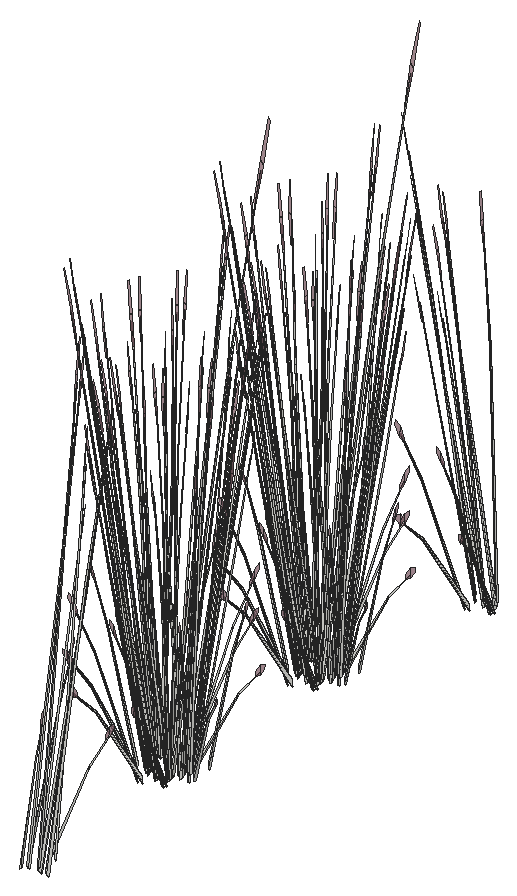
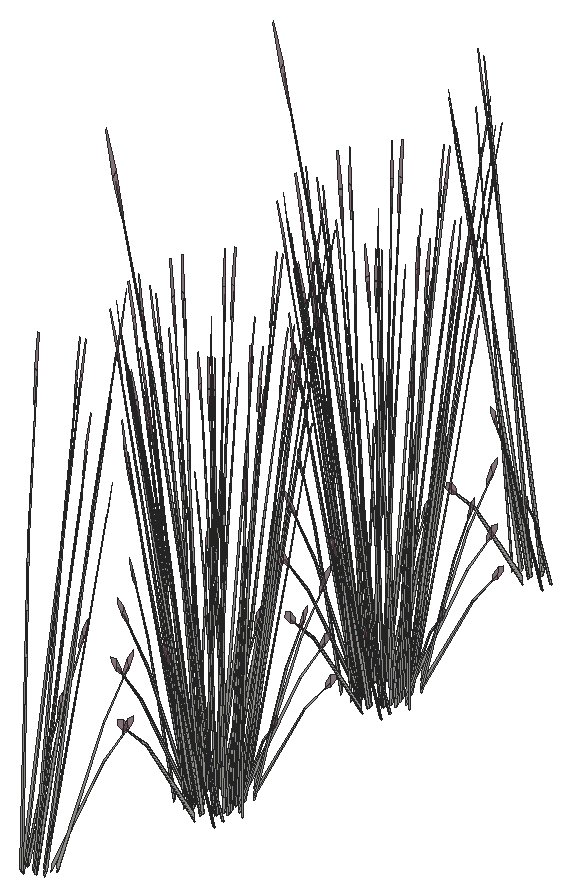
# SketchUp Ruby script. Lengths in inches.
U = 1.inch
M = Sketchup.active_model
def pt(a) = Geom::Point3d.new(a.map { |v| v * U })
def face(e, loops, mat)
  f = e.add_face(loops[0].map { |a| pt(a) })
  loops[1..].each { |l| e.add_face(l.map { |a| pt(a) }).erase! }
  f.material = f.back_material = mat if mat
  f
end
# faces: each face lists its corners as indices into pts; further lists are holes
def faces(e, pts, list, mat = nil) = list.each { |f| face(e, (f[0].is_a?(Array) ? f : [f]).map { |l| l.map { |i| pts[i] } }, mat) }
# xy, xz, yz: faces in a plane at the given z, y or x. An outline is a flat list of corners, or four numbers for a rectangle; further outlines are holes
def ring(l) = l.size == 4 ? [[l[0], l[1]], [l[2], l[1]], [l[2], l[3]], [l[0], l[3]]] : l.each_slice(2).to_a
def flat(e, list, mat, &to3) = list.each { |f| face(e, (f[0].is_a?(Array) ? f : [f]).map { |l| ring(l).map { |u, v| to3.(u, v) } }, mat) }
def xy(e, z, list, mat = nil) = flat(e, list, mat) { |x, y| [x, y, z] }
def xz(e, y, list, mat = nil) = flat(e, list, mat) { |x, z| [x, y, z] }
def yz(e, x, list, mat = nil) = flat(e, list, mat) { |y, z| [x, y, z] }
def lines(e, pts, list) = list.each { |a, b| e.add_line(pt(pts[a]), pt(pts[b])) }
# prism: a flat outline (further loops are holes) pulled along v
def prism(e, loops, v, mat = nil)
  f = face(e, loops, mat); d = Geom::Vector3d.new(v.map { |x| x * U })
  f.pushpull(f.normal.samedirection?(d) ? d.length : -d.length)
end
def box(e, o, s, mat = nil) = prism(e, [[o, [o[0] + s[0], o[1], o[2]], [o[0] + s[0], o[1] + s[1], o[2]], [o[0], o[1] + s[1], o[2]]]], [0, 0, s[2]], mat)
def at(x, y, z, deg = 0) = Geom::Transformation.translation(pt([x, y, z])) * Geom::Transformation.rotation(ORIGIN, Z_AXIS, deg.degrees)
def axes(o, x, y, z) = Geom::Transformation.new([*x, 0, *y, 0, *z, 0, *pt(o).to_a, 1])
def part(name) = M.definitions.add(name)
# library, detail: a bought-in or finely detailed component or shape, given as its bounding box
def library(name, o, s) = part(name).tap { |d| box(d.entities, o, s) }
def detail(e, o, s) = box(e.add_group.entities, o, s)
def put(e, d, t, mat = nil) = e.add_instance(d, t).tap { |i| i.material = mat if mat }
def group(e, t, mat = nil) = e.add_group.tap { |g| g.transformation = t; g.material = mat if mat }.entities
root = M.entities
M.materials.add("LightPink_Translucent").color = [144, 107, 117]
M.materials["LightPink_Translucent"].alpha = 0.75
c1 = part("blade")
p = [[2.15,0.21,22],[0,0.17,0],[0.09,0.45,0],[2.18,0.31,22],[2.29,0.31,22],[0.38,0.45,0],
  [2.48,0.24,33],[2.49,0.24,33],[2.48,0.22,33]]
faces(c1.entities,p,[[0,1,2,3],[4,5,2,3],[6,3,4,7],[8,0,3,6]])
c2 = part("seeds")
p = [[0.3,-0.1,1.38],[-0.01,-0.03,1.59],[-0.01,-0.03,0.03],[0.14,-0.07,-0.07],[0.29,-0.03,3],[0.15,0.01,3.11]]
faces(c2.entities,p,[[0,1,2,3],[1,0,4,5]],"LightPink_Translucent")
c3 = part("blade with seeds")
put(c3.entities,c1,at(0,0,0))
put(c3.entities,c2,axes([2.4,0.25,30.99],[1.5799,-0.05474,1.17369],[-0.12525,1.92788,0.29478],[-0.07173,-0.02425,1.56792]))
put(root,c3,axes([402.1875,258.22,5.65],[0.2439,-0.26754,-0.06488],[0.22348,0.29302,-0.29416],[0.01573,0.08303,0.97024]))
put(root,c3,axes([402.63,257.14,4.73],[-0.35104,0.10702,0.48003],[-0.06092,-0.41983,0.3958],[0.08256,0.12373,0.9933]))
put(root,c3,axes([401.67,257.27,4.73],[-0.26007,0.1585,0.0643],[-0.12729,-0.28902,0.50621],[0.02512,0.1274,0.77189]))
put(root,c3,axes([400.15,256.8125,4.72],[-0.00877,0.09229,1.74944],[0.24897,0.32105,-0.27667],[-0.06518,0.15182,0.14031]))
put(root,c3,axes([400.95,256.6,5.4],[0.3879,0.02311,-0.13498],[-0.0106,0.43749,-0.74919],[-0.02694,0.1685,1.13838]))
put(root,c3,axes([401.67,257.09,5.03],[0.34538,-0.21713,-0.1216],[0.16972,0.38536,-0.67495],[0.04557,0.16239,1.02557]))
put(root,c3,axes([401.77,257.23,5.0625],[-0.34777,-0.12192,0.53283],[0.11892,-0.40083,0.43934],[0.0209,0.15763,1.10256]))
put(root,c3,axes([400.125,257.76,4.71],[0.04004,-0.02816,1.77383],[0.33095,0.18728,-0.16761],[-0.00778,0.15594,0.31391]))
put(root,c3,axes([401.58,257.95,4.72],[0.04474,0.0751,1.74944],[0.36104,0.0295,-0.27667],[0.03631,0.16562,0.14031]))
put(root,c3,axes([399.37,272.02,4.72],[-0.05398,-0.06539,1.74944],[-0.36026,0.04145,-0.27667],[-0.0575,-0.15639,0.14031]))
put(root,c3,axes([400.98,272.82,4.72],[-0.00341,-0.09282,1.74944],[-0.28775,-0.26825,-0.27667],[0.04449,-0.16261,0.14031]))
put(root,c3,axes([400.91,272.49,4.71],[-0.03584,0.03562,1.77383],[-0.35118,-0.12018,-0.16761],[-0.01271,-0.15545,0.31391]))
put(root,c3,axes([399,271.81,4.71],[-0.00658,0.0559,1.77383],[-0.32474,0.20287,-0.16761],[-0.09556,-0.1037,0.31391]))
put(root,c3,axes([398.93,272.8,5.09],[0.39316,-0.11987,0.53763],[0.06823,0.47021,0.4433],[-0.09247,-0.13858,1.11249]))
put(root,c3,axes([399.81,272.89,4.73],[0.34777,0.12192,0.48003],[-0.11892,0.40083,0.3958],[-0.0209,-0.15763,0.9933]))
put(root,c3,axes([399.91,273.03,5.03],[-0.34538,0.21713,-0.1216],[-0.16972,-0.38536,-0.67495],[-0.04557,-0.16239,1.02557]))
put(root,c3,axes([400.63,273.52,5.03],[-0.3879,-0.02311,-0.1216],[0.0106,-0.43749,-0.67495],[0.02694,-0.1685,1.02557]))
put(root,c3,axes([399.91,272.86,4.73],[0.26007,-0.1585,0.0643],[0.12729,0.28902,0.50621],[-0.02512,-0.1274,0.77189]))
put(root,c3,axes([399.02,272.9,4.73],[0.16041,-0.29625,0.0643],[0.22843,0.17248,0.50621],[-0.07385,-0.09498,0.77189]))
put(root,c3,axes([399.8125,273.18,5.05],[-0.1064,0.35863,0.35414],[-0.31043,-0.1046,-0.4572],[-0.02846,-0.14439,0.87481]))
put(root,c3,axes([400.6,273.33,4.73],[0.25132,0.3182,0.48003],[-0.2669,0.27442,0.3958],[0.04636,-0.14929,0.9933]))
put(root,c3,axes([399.09,272.87,5.43],[-0.23555,0.44708,-0.13619],[-0.34112,-0.25757,-0.75594],[-0.11858,-0.12631,1.14864]))
put(root,c3,axes([400.7,273.36,4.73],[0.29004,0.02173,0.0643],[-0.00795,0.32812,0.50621],[0.03035,-0.12569,0.77189]))
put(root,c3,axes([400.48,273.59,5.05],[-0.23881,0.24554,0.35414],[-0.22606,-0.28036,-0.4572],[0.0344,-0.14245,0.87481]))
put(root,c3,axes([398.19,272.74,4.72],[-0.07594,-0.00329,1.74944],[-0.24177,0.32918,-0.27667],[-0.129,-0.06726,0.14031]))
put(root,c3,axes([401.05,274.38,5.03],[-0.32648,-0.25715,-0.1216],[0.18809,-0.3724,-0.67495],[0.09224,-0.12945,1.02557]))
put(root,c3,axes([399.07,273.24,5.05],[0.05451,0.37564,0.35414],[-0.31161,0.09919,-0.4572],[-0.0837,-0.10765,0.87481]))
put(root,c3,axes([398.13,273.49,5.09],[0.29147,-0.34417,0.53763],[0.25138,0.3655,0.4433],[-0.13675,-0.06349,1.11249]))
put(root,c3,axes([401.86,274.27,4.71],[-0.0461,-0.00354,1.77383],[-0.19143,-0.37951,-0.16761],[0.07688,-0.12478,0.31391]))
put(root,c3,axes([398.26,273.48,4.73],[0.01777,-0.35463,0.0643],[0.26836,0.00972,0.50621],[-0.1028,-0.03711,0.77189]))
put(root,c3,axes([400.9,274.35,5.05],[-0.30722,0.06665,0.35414],[-0.08112,-0.381,-0.4572],[0.08804,-0.10234,0.87481]))
put(root,c3,axes([401.17,274.28,4.73],[0.2423,0.19613,0.0643],[-0.14107,0.2793,0.50621],[0.07768,-0.0903,0.77189]))
put(root,c3,axes([401.11,274.2,4.73],[0.08753,0.42921,0.48003],[-0.34336,0.07449,0.3958],[0.1012,-0.10094,0.9933]))
put(root,c3,axes([402.03,274.72,4.72],[0.04898,-0.07104,1.74944],[-0.06269,-0.43574,-0.27667],[0.12289,-0.08262,0.14031]))
put(root,c3,axes([397.89,273.02,4.71],[0.02617,0.04654,1.77383],[-0.12614,0.41836,-0.16761],[-0.12775,0.00303,0.31391]))
put(root,c3,axes([398.44,273.75,5.05],[0.20082,0.29199,0.35414],[-0.2293,0.2764,-0.4572],[-0.1165,-0.04206,0.87481]))
put(root,c3,axes([398.39,273.5625,5.03],[-0.0189,0.47427,-0.1216],[-0.35781,-0.01296,-0.67495],[-0.13781,-0.03295,1.02557]))
put(root,c3,axes([401.07,275.38,5.03],[-0.17758,-0.42229,-0.1216],[0.31518,-0.20752,-0.67495],[0.13282,-0.05572,1.02557]))
put(root,c3,axes([400.94,275.26,5.05],[-0.29332,-0.1301,0.35414],[0.08555,-0.37955,-0.4572],[0.11809,-0.0348,0.87481]))
put(root,c3,axes([397.875,274.5625,4.73],[0.09971,-0.42522,0.48003],[0.32782,0.1454,0.3958],[-0.12892,0.02555,0.9933]))
put(root,c3,axes([397.85,274.45,4.73],[-0.12963,-0.31798,0.0643],[0.23638,-0.15564,0.50621],[-0.1042,0.03071,0.77189]))
put(root,c3,axes([401.21,275.375,4.73],[0.12963,0.31798,0.0643],[-0.23638,0.15564,0.50621],[0.1042,-0.03071,0.77189]))
put(root,c3,axes([401.18,275.26,4.73],[-0.09971,0.42522,0.48003],[-0.32782,-0.1454,0.3958],[0.12892,-0.02555,0.9933]))
put(root,c3,axes([398.11,274.57,5.05],[0.29332,0.1301,0.35414],[-0.08555,0.37955,-0.4572],[-0.11809,0.0348,0.87481]))
put(root,c3,axes([401.77,276.64,4.71],[-0.03191,-0.04083,1.77383],[0.06981,-0.43764,-0.16761],[0.12571,-0.02796,0.31391]))
put(root,c3,axes([397.62,274.86,4.72],[-0.05763,0.06055,1.74944],[0.0049,0.44239,-0.27667],[-0.13211,0.05753,0.14031]))
put(root,c3,axes([397.99,274.44,5.03],[0.17758,0.42229,-0.1216],[-0.31518,0.20752,-0.67495],[-0.13282,0.05572,1.02557]))
put(root,c3,axes([400.67,276.26,5.03],[0.0189,-0.47427,-0.1216],[0.35781,0.01296,-0.67495],[0.13781,0.03295,1.02557]))
put(root,c3,axes([400.61,276.07,5.05],[-0.20082,-0.29199,0.35414],[0.2293,-0.2764,-0.4572],[0.1165,0.04206,0.87481]))
put(root,c3,axes([400.98,275.98,4.72],[0.07571,-0.00789,1.74944],[0.20767,-0.36231,-0.27667],[0.13467,0.04783,0.14031]))
put(root,c3,axes([397.95,275.62,4.73],[-0.08753,-0.42921,0.48003],[0.34336,-0.07449,0.3958],[-0.1012,0.10094,0.9933]))
put(root,c3,axes([397.88,275.54,4.73],[-0.2423,-0.19613,0.0643],[0.14107,-0.2793,0.50621],[-0.07768,0.0903,0.77189]))
put(root,c3,axes([398.16,275.48,5.05],[0.30722,-0.06665,0.35414],[0.08112,0.381,-0.4572],[-0.08804,0.10234,0.87481]))
put(root,c3,axes([396.98,275.31,4.71],[0.04504,0.01251,1.77383],[0.13934,0.41205,-0.16761],[-0.0922,0.10815,0.31391]))
put(root,c3,axes([400.8,276.34,4.73],[-0.01777,0.35463,0.0643],[-0.26836,-0.00972,0.50621],[0.1028,0.03711,0.77189]))
put(root,c3,axes([400.82,276.23,4.73],[-0.26024,0.30729,0.48003],[-0.22444,-0.32634,0.3958],[0.1221,0.05668,0.9933]))
put(root,c3,axes([397.47,276.5625,5.65],[0.31145,0.12449,-0.06488],[-0.0958,0.38314,-0.29416],[-0.05094,0.05817,0.97024]))
put(root,c3,axes([399.99,276.58,5.05],[-0.05451,-0.37564,0.35414],[0.31161,-0.09919,-0.4572],[0.0837,0.10765,0.87481]))
put(root,c3,axes([400.2,274.42,4.47],[-0.30498,-0.24231,1.38283],[0.32203,-0.37727,0.59665],[0.0984,0.22736,1.33663]))
put(root,c3,axes([398,275.44,5.03],[0.32648,0.25715,-0.1216],[-0.18809,0.3724,-0.67495],[-0.09224,0.12945,1.02557]))
put(root,c3,axes([399.96,276.78,5.03],[0.21031,-0.39918,-0.1216],[0.30457,0.22997,-0.67495],[0.10587,0.11278,1.02557]))
put(root,c3,axes([398.58,276.24,5.05],[0.23881,-0.24554,0.35414],[0.22606,0.28036,-0.4572],[-0.0344,0.14245,0.87481]))
put(root,c3,axes([399.6875,277.11,4.71],[0.00104,-0.05646,1.77383],[0.30246,-0.2491,-0.16761],[0.10506,0.08891,0.31391]))
put(root,c3,axes([398.36,276.46,4.73],[-0.29004,-0.02173,0.0643],[0.00795,-0.32812,0.50621],[-0.03035,0.12569,0.77189]))
put(root,c3,axes([398.45,276.49,4.73],[-0.25132,-0.3182,0.48003],[0.2669,-0.27442,0.3958],[-0.04636,0.14929,0.9933]))
put(root,c3,axes([399.25,276.64,5.05],[0.1064,-0.35863,0.35414],[0.31043,0.1046,-0.4572],[0.02846,0.14439,0.87481]))
put(root,c3,axes([400.04,276.92,4.73],[-0.16041,0.29625,0.0643],[-0.22843,-0.17248,0.50621],[0.07385,0.09498,0.77189]))
put(root,c3,axes([399.67,277.92,5.65],[0.2439,-0.26754,-0.06488],[0.22348,0.29302,-0.29416],[0.01573,0.08303,0.97024]))
put(root,c3,axes([400.11,276.84,4.73],[-0.35104,0.10702,0.48003],[-0.06092,-0.41983,0.3958],[0.08256,0.12373,0.9933]))
put(root,c3,axes([399.15,276.97,4.73],[-0.26007,0.1585,0.0643],[-0.12729,-0.28902,0.50621],[0.02512,0.1274,0.77189]))
put(root,c3,axes([397.63,276.51,4.72],[-0.00877,0.09229,1.74944],[0.24897,0.32105,-0.27667],[-0.06518,0.15182,0.14031]))
put(root,c3,axes([398.43,276.31,5.4],[0.3879,0.02311,-0.13498],[-0.0106,0.43749,-0.74919],[-0.02694,0.1685,1.13838]))
put(root,c3,axes([399.14,276.79,5.03],[0.34538,-0.21713,-0.1216],[0.16972,0.38536,-0.67495],[0.04557,0.16239,1.02557]))
put(root,c3,axes([399.24,276.9375,5.0625],[-0.34777,-0.12192,0.53283],[0.11892,-0.40083,0.43934],[0.0209,0.15763,1.10256]))
put(root,c3,axes([397.6,277.46,4.71],[0.04004,-0.02816,1.77383],[0.33095,0.18728,-0.16761],[-0.00778,0.15594,0.31391]))
put(root,c3,axes([399.0625,277.66,4.72],[0.04474,0.0751,1.74944],[0.36104,0.0295,-0.27667],[0.03631,0.16562,0.14031]))
put(root,c3,axes([398.92,289.79,4.72],[-0.05398,-0.06539,1.74944],[-0.36026,0.04145,-0.27667],[-0.0575,-0.15639,0.14031]))
put(root,c3,axes([400.54,290.59,4.72],[-0.00341,-0.09282,1.74944],[-0.28775,-0.26825,-0.27667],[0.04449,-0.16261,0.14031]))
put(root,c3,axes([400.46,290.25,4.71],[-0.03584,0.03562,1.77383],[-0.35118,-0.12018,-0.16761],[-0.01271,-0.15545,0.31391]))
put(root,c3,axes([398.55,289.57,4.71],[-0.00658,0.0559,1.77383],[-0.32474,0.20287,-0.16761],[-0.09556,-0.1037,0.31391]))
put(root,c3,axes([398.48,290.5625,5.09],[0.39316,-0.11987,0.53763],[0.06823,0.47021,0.4433],[-0.09247,-0.13858,1.11249]))
put(root,c3,axes([399.37,290.65,4.73],[0.34777,0.12192,0.48003],[-0.11892,0.40083,0.3958],[-0.0209,-0.15763,0.9933]))
put(root,c3,axes([399.47,290.79,5.03],[-0.34538,0.21713,-0.1216],[-0.16972,-0.38536,-0.67495],[-0.04557,-0.16239,1.02557]))
put(root,c3,axes([400.1875,291.28,5.03],[-0.3879,-0.02311,-0.1216],[0.0106,-0.43749,-0.67495],[0.02694,-0.1685,1.02557]))
put(root,c3,axes([399.46,290.62,4.73],[0.26007,-0.1585,0.0643],[0.12729,0.28902,0.50621],[-0.02512,-0.1274,0.77189]))
put(root,c3,axes([398.57,290.67,4.73],[0.16041,-0.29625,0.0643],[0.22843,0.17248,0.50621],[-0.07385,-0.09498,0.77189]))
put(root,c3,axes([399.36,290.95,5.05],[-0.1064,0.35863,0.35414],[-0.31043,-0.1046,-0.4572],[-0.02846,-0.14439,0.87481]))
put(root,c3,axes([400.16,291.1,4.73],[0.25132,0.3182,0.48003],[-0.2669,0.27442,0.3958],[0.04636,-0.14929,0.9933]))
put(root,c3,axes([398.64,290.63,5.43],[-0.23555,0.44708,-0.13619],[-0.34112,-0.25757,-0.75594],[-0.11858,-0.12631,1.14864]))
put(root,c3,axes([400.25,291.13,4.73],[0.29004,0.02173,0.0643],[-0.00795,0.32812,0.50621],[0.03035,-0.12569,0.77189]))
put(root,c3,axes([400.03,291.35,5.05],[-0.23881,0.24554,0.35414],[-0.22606,-0.28036,-0.4572],[0.0344,-0.14245,0.87481]))
put(root,c3,axes([397.74,290.51,4.72],[-0.07594,-0.00329,1.74944],[-0.24177,0.32918,-0.27667],[-0.129,-0.06726,0.14031]))
put(root,c3,axes([400.61,292.14,5.03],[-0.32648,-0.25715,-0.1216],[0.18809,-0.3724,-0.67495],[0.09224,-0.12945,1.02557]))
put(root,c3,axes([398.62,291.01,5.05],[0.05451,0.37564,0.35414],[-0.31161,0.09919,-0.4572],[-0.0837,-0.10765,0.87481]))
put(root,c3,axes([397.68,291.25,5.09],[0.29147,-0.34417,0.53763],[0.25138,0.3655,0.4433],[-0.13675,-0.06349,1.11249]))
put(root,c3,axes([401.41,292.03,4.71],[-0.0461,-0.00354,1.77383],[-0.19143,-0.37951,-0.16761],[0.07688,-0.12478,0.31391]))
put(root,c3,axes([397.82,291.25,4.73],[0.01777,-0.35463,0.0643],[0.26836,0.00972,0.50621],[-0.1028,-0.03711,0.77189]))
put(root,c3,axes([400.45,292.11,5.05],[-0.30722,0.06665,0.35414],[-0.08112,-0.381,-0.4572],[0.08804,-0.10234,0.87481]))
put(root,c3,axes([400.73,292.05,4.73],[0.2423,0.19613,0.0643],[-0.14107,0.2793,0.50621],[0.07768,-0.0903,0.77189]))
put(root,c3,axes([400.66,291.97,4.73],[0.08753,0.42921,0.48003],[-0.34336,0.07449,0.3958],[0.1012,-0.10094,0.9933]))
put(root,c3,axes([401.59,292.49,4.72],[0.04898,-0.07104,1.74944],[-0.06269,-0.43574,-0.27667],[0.12289,-0.08262,0.14031]))
put(root,c3,axes([397.45,290.78,4.71],[0.02617,0.04654,1.77383],[-0.12614,0.41836,-0.16761],[-0.12775,0.00303,0.31391]))
put(root,c3,axes([398,291.51,5.05],[0.20082,0.29199,0.35414],[-0.2293,0.2764,-0.4572],[-0.1165,-0.04206,0.87481]))
put(root,c3,axes([397.94,291.33,5.03],[-0.0189,0.47427,-0.1216],[-0.35781,-0.01296,-0.67495],[-0.13781,-0.03295,1.02557]))
put(root,c3,axes([400.62,293.15,5.03],[-0.17758,-0.42229,-0.1216],[0.31518,-0.20752,-0.67495],[0.13282,-0.05572,1.02557]))
put(root,c3,axes([400.5,293.02,5.05],[-0.29332,-0.1301,0.35414],[0.08555,-0.37955,-0.4572],[0.11809,-0.0348,0.87481]))
put(root,c3,axes([397.43,292.33,4.73],[0.09971,-0.42522,0.48003],[0.32782,0.1454,0.3958],[-0.12892,0.02555,0.9933]))
put(root,c3,axes([397.4,292.21,4.73],[-0.12963,-0.31798,0.0643],[0.23638,-0.15564,0.50621],[-0.1042,0.03071,0.77189]))
put(root,c3,axes([400.76,293.14,4.73],[0.12963,0.31798,0.0643],[-0.23638,0.15564,0.50621],[0.1042,-0.03071,0.77189]))
put(root,c3,axes([400.74,293.03,4.73],[-0.09971,0.42522,0.48003],[-0.32782,-0.1454,0.3958],[0.12892,-0.02555,0.9933]))
put(root,c3,axes([397.67,292.33,5.05],[0.29332,0.1301,0.35414],[-0.08555,0.37955,-0.4572],[-0.11809,0.0348,0.87481]))
put(root,c3,axes([401.33,294.4,4.71],[-0.03191,-0.04083,1.77383],[0.06981,-0.43764,-0.16761],[0.12571,-0.02796,0.31391]))
put(root,c3,axes([397.17,292.625,4.72],[-0.05763,0.06055,1.74944],[0.0049,0.44239,-0.27667],[-0.13211,0.05753,0.14031]))
put(root,c3,axes([397.54,292.2,5.03],[0.17758,0.42229,-0.1216],[-0.31518,0.20752,-0.67495],[-0.13282,0.05572,1.02557]))
put(root,c3,axes([400.22,294.02,5.03],[0.0189,-0.47427,-0.1216],[0.35781,0.01296,-0.67495],[0.13781,0.03295,1.02557]))
put(root,c3,axes([400.17,293.84,5.05],[-0.20082,-0.29199,0.35414],[0.2293,-0.2764,-0.4572],[0.1165,0.04206,0.87481]))
put(root,c3,axes([400.53,293.74,4.72],[0.07571,-0.00789,1.74944],[0.20767,-0.36231,-0.27667],[0.13467,0.04783,0.14031]))
put(root,c3,axes([397.51,293.39,4.73],[-0.08753,-0.42921,0.48003],[0.34336,-0.07449,0.3958],[-0.1012,0.10094,0.9933]))
put(root,c3,axes([397.4375,293.3,4.73],[-0.2423,-0.19613,0.0643],[0.14107,-0.2793,0.50621],[-0.07768,0.0903,0.77189]))
put(root,c3,axes([397.72,293.24,5.05],[0.30722,-0.06665,0.35414],[0.08112,0.381,-0.4572],[-0.08804,0.10234,0.87481]))
put(root,c3,axes([396.53,293.07,4.71],[0.04504,0.01251,1.77383],[0.13934,0.41205,-0.16761],[-0.0922,0.10815,0.31391]))
put(root,c3,axes([400.35,294.1,4.73],[-0.01777,0.35463,0.0643],[-0.26836,-0.00972,0.50621],[0.1028,0.03711,0.77189]))
put(root,c3,axes([400.375,293.99,4.73],[-0.26024,0.30729,0.48003],[-0.22444,-0.32634,0.3958],[0.1221,0.05668,0.9933]))
put(root,c3,axes([397.02,294.32,5.65],[0.31145,0.12449,-0.06488],[-0.0958,0.38314,-0.29416],[-0.05094,0.05817,0.97024]))
put(root,c3,axes([399.55,294.35,5.05],[-0.05451,-0.37564,0.35414],[0.31161,-0.09919,-0.4572],[0.0837,0.10765,0.87481]))
put(root,c3,axes([399.76,292.19,4.47],[-0.30498,-0.24231,1.38283],[0.32203,-0.37727,0.59665],[0.0984,0.22736,1.33663]))
put(root,c3,axes([397.56,293.21,5.03],[0.32648,0.25715,-0.1216],[-0.18809,0.3724,-0.67495],[-0.09224,0.12945,1.02557]))
put(root,c3,axes([399.52,294.54,5.03],[0.21031,-0.39918,-0.1216],[0.30457,0.22997,-0.67495],[0.10587,0.11278,1.02557]))
put(root,c3,axes([398.13,294,5.05],[0.23881,-0.24554,0.35414],[0.22606,0.28036,-0.4572],[-0.0344,0.14245,0.87481]))
put(root,c3,axes([399.24,294.87,4.71],[0.00104,-0.05646,1.77383],[0.30246,-0.2491,-0.16761],[0.10506,0.08891,0.31391]))
put(root,c3,axes([397.92,294.22,4.73],[-0.29004,-0.02173,0.0643],[0.00795,-0.32812,0.50621],[-0.03035,0.12569,0.77189]))
put(root,c3,axes([398.01,294.25,4.73],[-0.25132,-0.3182,0.48003],[0.2669,-0.27442,0.3958],[-0.04636,0.14929,0.9933]))
put(root,c3,axes([398.8,294.41,5.05],[0.1064,-0.35863,0.35414],[0.31043,0.1046,-0.4572],[0.02846,0.14439,0.87481]))
put(root,c3,axes([399.6,294.6875,4.73],[-0.16041,0.29625,0.0643],[-0.22843,-0.17248,0.50621],[0.07385,0.09498,0.77189]))
put(root,c3,axes([399.22,295.69,5.65],[0.2439,-0.26754,-0.06488],[0.22348,0.29302,-0.29416],[0.01573,0.08303,0.97024]))
put(root,c3,axes([399.66,294.6,4.73],[-0.35104,0.10702,0.48003],[-0.06092,-0.41983,0.3958],[0.08256,0.12373,0.9933]))
put(root,c3,axes([398.71,294.73,4.73],[-0.26007,0.1585,0.0643],[-0.12729,-0.28902,0.50621],[0.02512,0.1274,0.77189]))
put(root,c3,axes([397.18,294.28,4.72],[-0.00877,0.09229,1.74944],[0.24897,0.32105,-0.27667],[-0.06518,0.15182,0.14031]))
put(root,c3,axes([397.98,294.07,5.4],[0.3879,0.02311,-0.13498],[-0.0106,0.43749,-0.74919],[-0.02694,0.1685,1.13838]))
put(root,c3,axes([398.7,294.56,5.03],[0.34538,-0.21713,-0.1216],[0.16972,0.38536,-0.67495],[0.04557,0.16239,1.02557]))
put(root,c3,axes([398.8,294.7,5.0625],[-0.34777,-0.12192,0.53283],[0.11892,-0.40083,0.43934],[0.0209,0.15763,1.10256]))
put(root,c3,axes([397.16,295.22,4.71],[0.04004,-0.02816,1.77383],[0.33095,0.18728,-0.16761],[-0.00778,0.15594,0.31391]))
put(root,c3,axes([398.62,295.42,4.72],[0.04474,0.0751,1.74944],[0.36104,0.0295,-0.27667],[0.03631,0.16562,0.14031]))
put(root,c3,axes([401.89,306.35,4.72],[-0.05398,-0.06539,1.74944],[-0.36026,0.04145,-0.27667],[-0.0575,-0.15639,0.14031]))
put(root,c3,axes([403.51,307.15,4.72],[-0.00341,-0.09282,1.74944],[-0.28775,-0.26825,-0.27667],[0.04449,-0.16261,0.14031]))
put(root,c3,axes([403.43,306.82,4.71],[-0.03584,0.03562,1.77383],[-0.35118,-0.12018,-0.16761],[-0.01271,-0.15545,0.31391]))
put(root,c3,axes([401.52,306.14,4.71],[-0.00658,0.0559,1.77383],[-0.32474,0.20287,-0.16761],[-0.09556,-0.1037,0.31391]))
put(root,c3,axes([401.45,307.13,5.09],[0.39316,-0.11987,0.53763],[0.06823,0.47021,0.4433],[-0.09247,-0.13858,1.11249]))
put(root,c3,axes([402.34,307.22,4.73],[0.34777,0.12192,0.48003],[-0.11892,0.40083,0.3958],[-0.0209,-0.15763,0.9933]))
put(root,c3,axes([402.4375,307.36,5.03],[-0.34538,0.21713,-0.1216],[-0.16972,-0.38536,-0.67495],[-0.04557,-0.16239,1.02557]))
put(root,c3,axes([403.15,307.85,5.03],[-0.3879,-0.02311,-0.1216],[0.0106,-0.43749,-0.67495],[0.02694,-0.1685,1.02557]))
put(root,c3,axes([402.43,307.18,4.73],[0.26007,-0.1585,0.0643],[0.12729,0.28902,0.50621],[-0.02512,-0.1274,0.77189]))
put(root,c3,axes([401.54,307.23,4.73],[0.16041,-0.29625,0.0643],[0.22843,0.17248,0.50621],[-0.07385,-0.09498,0.77189]))
put(root,c3,axes([402.33,307.51,5.05],[-0.1064,0.35863,0.35414],[-0.31043,-0.1046,-0.4572],[-0.02846,-0.14439,0.87481]))
put(root,c3,axes([403.125,307.66,4.73],[0.25132,0.3182,0.48003],[-0.2669,0.27442,0.3958],[0.04636,-0.14929,0.9933]))
